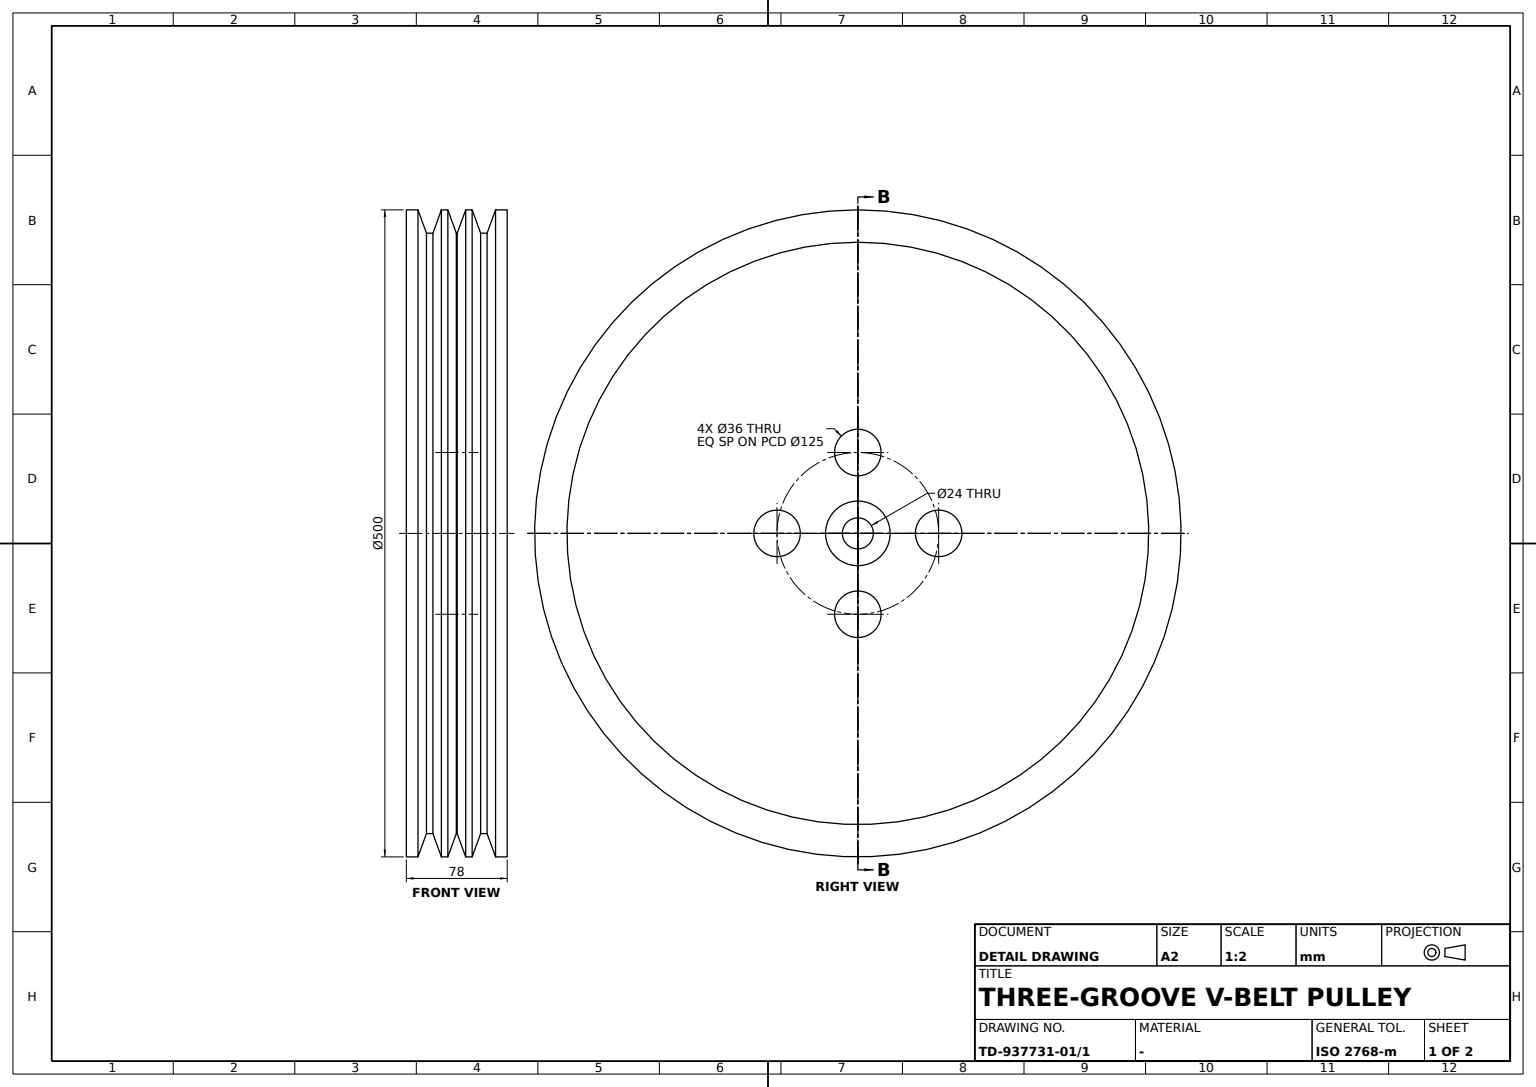
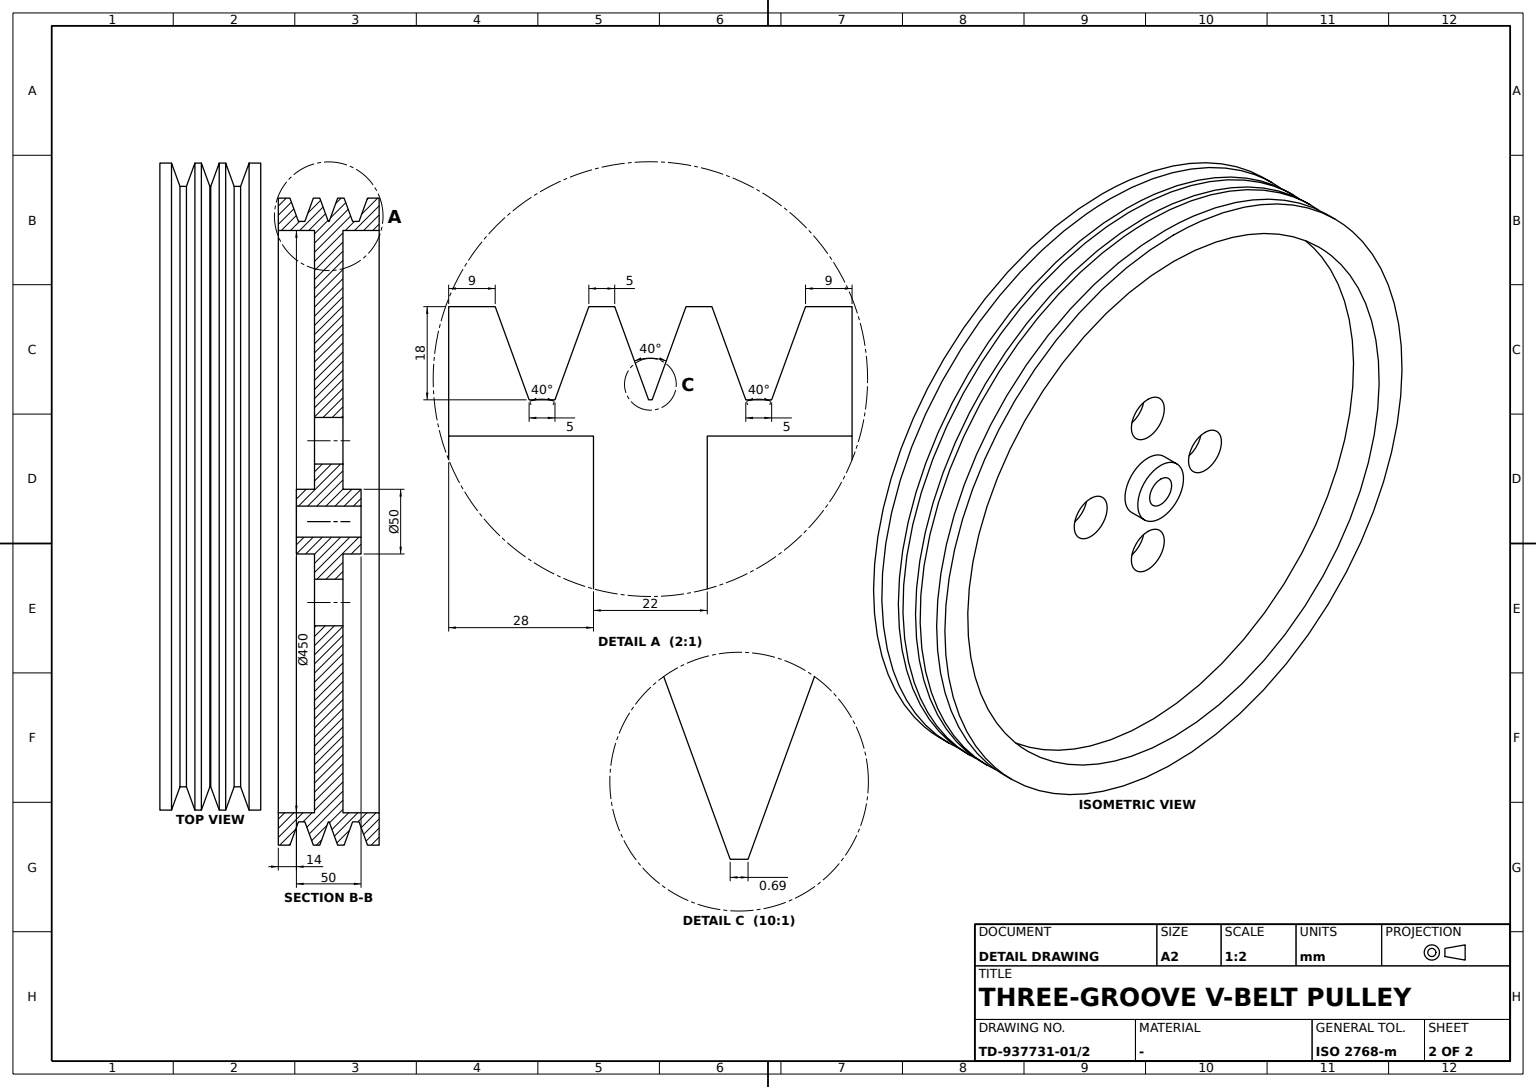
ISO-10303-21;
HEADER;
FILE_DESCRIPTION((''),'2;1');
FILE_NAME('','',(''),(''),'','','');
FILE_SCHEMA(('AUTOMOTIVE_DESIGN'));
ENDSEC;
DATA;
#1=APPLICATION_CONTEXT('');
#2=PRODUCT_CONTEXT('',#1,'mechanical');
#3=PRODUCT('','','',(#2));
#4=PRODUCT_DEFINITION_FORMATION('','',#3);
#5=PRODUCT_DEFINITION_CONTEXT('',#1,'design');
#6=PRODUCT_DEFINITION('','',#4,#5);
#7=PRODUCT_DEFINITION_SHAPE('','',#6);
#8=(LENGTH_UNIT()NAMED_UNIT(*)SI_UNIT(.MILLI.,.METRE.));
#9=(NAMED_UNIT(*)PLANE_ANGLE_UNIT()SI_UNIT($,.RADIAN.));
#10=(NAMED_UNIT(*)SI_UNIT($,.STERADIAN.)SOLID_ANGLE_UNIT());
#11=UNCERTAINTY_MEASURE_WITH_UNIT(LENGTH_MEASURE(0.005),#8,'distance_accuracy_value','');
#12=(GEOMETRIC_REPRESENTATION_CONTEXT(3)GLOBAL_UNCERTAINTY_ASSIGNED_CONTEXT((#11))GLOBAL_UNIT_ASSIGNED_CONTEXT((#8,#9,#10))REPRESENTATION_CONTEXT('',''));
#13=CARTESIAN_POINT('',(0.,6.897072,250.));
#14=VERTEX_POINT('',#13);
#15=CARTESIAN_POINT('',(0.,6.897072,0.));
#16=DIRECTION('',(0.,1.,0.));
#17=DIRECTION('',(0.,0.,1.));
#18=AXIS2_PLACEMENT_3D('',#15,#16,#17);
#19=CIRCLE('',#18,250.);
#20=EDGE_CURVE('',#14,#14,#19,.T.);
#21=ORIENTED_EDGE('',*,*,#20,.F.);
#22=EDGE_LOOP('',(#21));
#23=FACE_BOUND('',#22,.T.);
#24=CARTESIAN_POINT('',(0.,0.345607,232.));
#25=VERTEX_POINT('',#24);
#26=CARTESIAN_POINT('',(0.,0.345607,0.));
#27=AXIS2_PLACEMENT_3D('',#26,#16,#17);
#28=CIRCLE('',#27,232.);
#29=EDGE_CURVE('',#25,#25,#28,.T.);
#30=ORIENTED_EDGE('',*,*,#29,.T.);
#31=EDGE_LOOP('',(#30));
#32=FACE_BOUND('',#31,.T.);
#33=DIRECTION('',(1.,0.,0.));
#34=AXIS2_PLACEMENT_3D('',#26,#16,#33);
#35=CONICAL_SURFACE('',#34,232.,1.221730476);
#36=ADVANCED_FACE('',(#23,#32),#35,.T.);
#37=CARTESIAN_POINT('',(0.,25.,12.));
#38=VERTEX_POINT('',#37);
#39=CARTESIAN_POINT('',(0.,25.,0.));
#40=AXIS2_PLACEMENT_3D('',#39,#16,#17);
#41=CIRCLE('',#40,12.);
#42=EDGE_CURVE('',#38,#38,#41,.T.);
#43=ORIENTED_EDGE('',*,*,#42,.F.);
#44=EDGE_LOOP('',(#43));
#45=FACE_BOUND('',#44,.T.);
#46=CARTESIAN_POINT('',(0.,25.,25.));
#47=VERTEX_POINT('',#46);
#48=CIRCLE('',#40,25.);
#49=EDGE_CURVE('',#47,#47,#48,.T.);
#50=ORIENTED_EDGE('',*,*,#49,.T.);
#51=EDGE_LOOP('',(#50));
#52=FACE_BOUND('',#51,.T.);
#53=AXIS2_PLACEMENT_3D('',#46,#16,#33);
#54=PLANE('',#53);
#55=ADVANCED_FACE('',(#45,#52),#54,.T.);
#56=CARTESIAN_POINT('',(0.,18.448536,-232.));
#57=VERTEX_POINT('',#56);
#58=CARTESIAN_POINT('',(0.,18.448536,0.));
#59=DIRECTION('',(0.,-1.,0.));
#60=DIRECTION('',(0.,0.,-1.));
#61=AXIS2_PLACEMENT_3D('',#58,#59,#60);
#62=CIRCLE('',#61,232.);
#63=EDGE_CURVE('',#57,#57,#62,.F.);
#64=ORIENTED_EDGE('',*,*,#63,.F.);
#65=EDGE_LOOP('',(#64));
#66=FACE_BOUND('',#65,.T.);
#67=CARTESIAN_POINT('',(0.,11.897072,-250.));
#68=VERTEX_POINT('',#67);
#69=CARTESIAN_POINT('',(0.,11.897072,0.));
#70=AXIS2_PLACEMENT_3D('',#69,#59,#60);
#71=CIRCLE('',#70,250.);
#72=EDGE_CURVE('',#68,#68,#71,.F.);
#73=ORIENTED_EDGE('',*,*,#72,.T.);
#74=EDGE_LOOP('',(#73));
#75=FACE_BOUND('',#74,.T.);
#76=AXIS2_PLACEMENT_3D('',#58,#59,#33);
#77=CONICAL_SURFACE('',#76,232.,1.221730476);
#78=ADVANCED_FACE('',(#66,#75),#77,.T.);
#79=CARTESIAN_POINT('',(0.,30.,250.));
#80=VERTEX_POINT('',#79);
#81=CARTESIAN_POINT('',(0.,30.,0.));
#82=AXIS2_PLACEMENT_3D('',#81,#16,#17);
#83=CIRCLE('',#82,250.);
#84=EDGE_CURVE('',#80,#80,#83,.T.);
#85=ORIENTED_EDGE('',*,*,#84,.T.);
#86=EDGE_LOOP('',(#85));
#87=FACE_BOUND('',#86,.T.);
#88=CARTESIAN_POINT('',(0.,39.,250.));
#89=VERTEX_POINT('',#88);
#90=CARTESIAN_POINT('',(0.,39.,0.));
#91=AXIS2_PLACEMENT_3D('',#90,#16,#17);
#92=CIRCLE('',#91,250.);
#93=EDGE_CURVE('',#89,#89,#92,.T.);
#94=ORIENTED_EDGE('',*,*,#93,.F.);
#95=EDGE_LOOP('',(#94));
#96=FACE_BOUND('',#95,.T.);
#97=CARTESIAN_POINT('',(0.,0.,0.));
#98=AXIS2_PLACEMENT_3D('',#97,#16,#33);
#99=CYLINDRICAL_SURFACE('',#98,250.);
#100=ADVANCED_FACE('',(#87,#96),#99,.T.);
#101=ORIENTED_EDGE('',*,*,#42,.T.);
#102=EDGE_LOOP('',(#101));
#103=FACE_BOUND('',#102,.T.);
#104=CARTESIAN_POINT('',(0.,-25.,12.));
#105=VERTEX_POINT('',#104);
#106=CARTESIAN_POINT('',(0.,-25.,0.));
#107=AXIS2_PLACEMENT_3D('',#106,#16,#17);
#108=CIRCLE('',#107,12.);
#109=EDGE_CURVE('',#105,#105,#108,.T.);
#110=ORIENTED_EDGE('',*,*,#109,.F.);
#111=EDGE_LOOP('',(#110));
#112=FACE_BOUND('',#111,.T.);
#113=CYLINDRICAL_SURFACE('',#98,12.);
#114=ADVANCED_FACE('',(#103,#112),#113,.F.);
#115=CARTESIAN_POINT('',(0.,-11.,225.));
#116=VERTEX_POINT('',#115);
#117=CARTESIAN_POINT('',(0.,-11.,0.));
#118=AXIS2_PLACEMENT_3D('',#117,#16,#17);
#119=CIRCLE('',#118,225.);
#120=EDGE_CURVE('',#116,#116,#119,.T.);
#121=ORIENTED_EDGE('',*,*,#120,.T.);
#122=EDGE_LOOP('',(#121));
#123=FACE_BOUND('',#122,.T.);
#124=CARTESIAN_POINT('',(0.,-39.,225.));
#125=VERTEX_POINT('',#124);
#126=CARTESIAN_POINT('',(0.,-39.,0.));
#127=AXIS2_PLACEMENT_3D('',#126,#16,#17);
#128=CIRCLE('',#127,225.);
#129=EDGE_CURVE('',#125,#125,#128,.T.);
#130=ORIENTED_EDGE('',*,*,#129,.F.);
#131=EDGE_LOOP('',(#130));
#132=FACE_BOUND('',#131,.T.);
#133=CYLINDRICAL_SURFACE('',#98,225.);
#134=ADVANCED_FACE('',(#123,#132),#133,.F.);
#135=CARTESIAN_POINT('',(0.,-18.448536,232.));
#136=VERTEX_POINT('',#135);
#137=CARTESIAN_POINT('',(0.,-18.448536,0.));
#138=AXIS2_PLACEMENT_3D('',#137,#16,#17);
#139=CIRCLE('',#138,232.);
#140=EDGE_CURVE('',#136,#136,#139,.T.);
#141=ORIENTED_EDGE('',*,*,#140,.T.);
#142=EDGE_LOOP('',(#141));
#143=FACE_BOUND('',#142,.T.);
#144=CARTESIAN_POINT('',(0.,-11.897072,250.));
#145=VERTEX_POINT('',#144);
#146=CARTESIAN_POINT('',(0.,-11.897072,0.));
#147=AXIS2_PLACEMENT_3D('',#146,#16,#17);
#148=CIRCLE('',#147,250.);
#149=EDGE_CURVE('',#145,#145,#148,.T.);
#150=ORIENTED_EDGE('',*,*,#149,.F.);
#151=EDGE_LOOP('',(#150));
#152=FACE_BOUND('',#151,.T.);
#153=AXIS2_PLACEMENT_3D('',#137,#16,#33);
#154=CONICAL_SURFACE('',#153,232.,1.221730476);
#155=ADVANCED_FACE('',(#143,#152),#154,.T.);
#156=CARTESIAN_POINT('',(0.,-30.,-250.));
#157=VERTEX_POINT('',#156);
#158=CARTESIAN_POINT('',(0.,-30.,0.));
#159=AXIS2_PLACEMENT_3D('',#158,#59,#60);
#160=CIRCLE('',#159,250.);
#161=EDGE_CURVE('',#157,#157,#160,.F.);
#162=ORIENTED_EDGE('',*,*,#161,.T.);
#163=EDGE_LOOP('',(#162));
#164=FACE_BOUND('',#163,.T.);
#165=CARTESIAN_POINT('',(0.,-23.448536,-232.));
#166=VERTEX_POINT('',#165);
#167=CARTESIAN_POINT('',(0.,-23.448536,0.));
#168=AXIS2_PLACEMENT_3D('',#167,#59,#60);
#169=CIRCLE('',#168,232.);
#170=EDGE_CURVE('',#166,#166,#169,.F.);
#171=ORIENTED_EDGE('',*,*,#170,.F.);
#172=EDGE_LOOP('',(#171));
#173=FACE_BOUND('',#172,.T.);
#174=AXIS2_PLACEMENT_3D('',#167,#59,#33);
#175=CONICAL_SURFACE('',#174,232.,1.221730476);
#176=ADVANCED_FACE('',(#164,#173),#175,.T.);
#177=CARTESIAN_POINT('',(0.,-0.345607,-232.));
#178=VERTEX_POINT('',#177);
#179=CARTESIAN_POINT('',(0.,-0.345607,0.));
#180=AXIS2_PLACEMENT_3D('',#179,#59,#60);
#181=CIRCLE('',#180,232.);
#182=EDGE_CURVE('',#178,#178,#181,.F.);
#183=ORIENTED_EDGE('',*,*,#182,.F.);
#184=EDGE_LOOP('',(#183));
#185=FACE_BOUND('',#184,.T.);
#186=CARTESIAN_POINT('',(0.,-6.897072,-250.));
#187=VERTEX_POINT('',#186);
#188=CARTESIAN_POINT('',(0.,-6.897072,0.));
#189=AXIS2_PLACEMENT_3D('',#188,#59,#60);
#190=CIRCLE('',#189,250.);
#191=EDGE_CURVE('',#187,#187,#190,.F.);
#192=ORIENTED_EDGE('',*,*,#191,.T.);
#193=EDGE_LOOP('',(#192));
#194=FACE_BOUND('',#193,.T.);
#195=AXIS2_PLACEMENT_3D('',#179,#59,#33);
#196=CONICAL_SURFACE('',#195,232.,1.221730476);
#197=ADVANCED_FACE('',(#185,#194),#196,.T.);
#198=CARTESIAN_POINT('',(0.,-11.,-44.5));
#199=VERTEX_POINT('',#198);
#200=CARTESIAN_POINT('',(0.,-11.,-62.5));
#201=AXIS2_PLACEMENT_3D('',#200,#16,#17);
#202=CIRCLE('',#201,18.);
#203=EDGE_CURVE('',#199,#199,#202,.T.);
#204=ORIENTED_EDGE('',*,*,#203,.F.);
#205=EDGE_LOOP('',(#204));
#206=FACE_BOUND('',#205,.T.);
#207=CARTESIAN_POINT('',(0.,11.,-44.5));
#208=VERTEX_POINT('',#207);
#209=CARTESIAN_POINT('',(0.,11.,-62.5));
#210=AXIS2_PLACEMENT_3D('',#209,#16,#17);
#211=CIRCLE('',#210,18.);
#212=EDGE_CURVE('',#208,#208,#211,.T.);
#213=ORIENTED_EDGE('',*,*,#212,.T.);
#214=EDGE_LOOP('',(#213));
#215=FACE_BOUND('',#214,.T.);
#216=CARTESIAN_POINT('',(0.,-32.5,-62.5));
#217=DIRECTION('',(-1.,0.,0.));
#218=AXIS2_PLACEMENT_3D('',#216,#16,#217);
#219=CYLINDRICAL_SURFACE('',#218,18.);
#220=ADVANCED_FACE('',(#206,#215),#219,.F.);
#221=CARTESIAN_POINT('',(0.,11.,25.));
#222=VERTEX_POINT('',#221);
#223=CARTESIAN_POINT('',(0.,11.,0.));
#224=AXIS2_PLACEMENT_3D('',#223,#16,#17);
#225=CIRCLE('',#224,25.);
#226=EDGE_CURVE('',#222,#222,#225,.T.);
#227=ORIENTED_EDGE('',*,*,#226,.T.);
#228=EDGE_LOOP('',(#227));
#229=FACE_BOUND('',#228,.T.);
#230=ORIENTED_EDGE('',*,*,#49,.F.);
#231=EDGE_LOOP('',(#230));
#232=FACE_BOUND('',#231,.T.);
#233=CYLINDRICAL_SURFACE('',#98,25.);
#234=ADVANCED_FACE('',(#229,#232),#233,.T.);
#235=ORIENTED_EDGE('',*,*,#84,.F.);
#236=EDGE_LOOP('',(#235));
#237=FACE_BOUND('',#236,.T.);
#238=CARTESIAN_POINT('',(0.,23.448536,232.));
#239=VERTEX_POINT('',#238);
#240=CARTESIAN_POINT('',(0.,23.448536,0.));
#241=AXIS2_PLACEMENT_3D('',#240,#16,#17);
#242=CIRCLE('',#241,232.);
#243=EDGE_CURVE('',#239,#239,#242,.T.);
#244=ORIENTED_EDGE('',*,*,#243,.T.);
#245=EDGE_LOOP('',(#244));
#246=FACE_BOUND('',#245,.T.);
#247=AXIS2_PLACEMENT_3D('',#240,#16,#33);
#248=CONICAL_SURFACE('',#247,232.,1.221730476);
#249=ADVANCED_FACE('',(#237,#246),#248,.T.);
#250=CARTESIAN_POINT('',(-62.5,11.,18.));
#251=VERTEX_POINT('',#250);
#252=CARTESIAN_POINT('',(-62.5,11.,0.));
#253=AXIS2_PLACEMENT_3D('',#252,#16,#17);
#254=CIRCLE('',#253,18.);
#255=EDGE_CURVE('',#251,#251,#254,.T.);
#256=ORIENTED_EDGE('',*,*,#255,.T.);
#257=EDGE_LOOP('',(#256));
#258=FACE_BOUND('',#257,.T.);
#259=CARTESIAN_POINT('',(-62.5,-11.,18.));
#260=VERTEX_POINT('',#259);
#261=CARTESIAN_POINT('',(-62.5,-11.,0.));
#262=AXIS2_PLACEMENT_3D('',#261,#16,#17);
#263=CIRCLE('',#262,18.);
#264=EDGE_CURVE('',#260,#260,#263,.T.);
#265=ORIENTED_EDGE('',*,*,#264,.F.);
#266=EDGE_LOOP('',(#265));
#267=FACE_BOUND('',#266,.T.);
#268=CARTESIAN_POINT('',(-62.5,-32.5,0.));
#269=AXIS2_PLACEMENT_3D('',#268,#16,#217);
#270=CYLINDRICAL_SURFACE('',#269,18.);
#271=ADVANCED_FACE('',(#258,#267),#270,.F.);
#272=ORIENTED_EDGE('',*,*,#20,.T.);
#273=EDGE_LOOP('',(#272));
#274=FACE_BOUND('',#273,.T.);
#275=ORIENTED_EDGE('',*,*,#72,.F.);
#276=EDGE_LOOP('',(#275));
#277=FACE_BOUND('',#276,.T.);
#278=ADVANCED_FACE('',(#274,#277),#99,.T.);
#279=CARTESIAN_POINT('',(0.,11.,225.));
#280=VERTEX_POINT('',#279);
#281=CIRCLE('',#224,225.);
#282=EDGE_CURVE('',#280,#280,#281,.T.);
#283=ORIENTED_EDGE('',*,*,#282,.T.);
#284=EDGE_LOOP('',(#283));
#285=FACE_BOUND('',#284,.T.);
#286=CARTESIAN_POINT('',(62.5,11.,18.));
#287=VERTEX_POINT('',#286);
#288=CARTESIAN_POINT('',(62.5,11.,0.));
#289=AXIS2_PLACEMENT_3D('',#288,#16,#17);
#290=CIRCLE('',#289,18.);
#291=EDGE_CURVE('',#287,#287,#290,.T.);
#292=ORIENTED_EDGE('',*,*,#291,.F.);
#293=EDGE_LOOP('',(#292));
#294=FACE_BOUND('',#293,.T.);
#295=CARTESIAN_POINT('',(0.,11.,80.5));
#296=VERTEX_POINT('',#295);
#297=CARTESIAN_POINT('',(0.,11.,62.5));
#298=AXIS2_PLACEMENT_3D('',#297,#16,#17);
#299=CIRCLE('',#298,18.);
#300=EDGE_CURVE('',#296,#296,#299,.T.);
#301=ORIENTED_EDGE('',*,*,#300,.F.);
#302=EDGE_LOOP('',(#301));
#303=FACE_BOUND('',#302,.T.);
#304=ORIENTED_EDGE('',*,*,#212,.F.);
#305=EDGE_LOOP('',(#304));
#306=FACE_BOUND('',#305,.T.);
#307=ORIENTED_EDGE('',*,*,#255,.F.);
#308=EDGE_LOOP('',(#307));
#309=FACE_BOUND('',#308,.T.);
#310=ORIENTED_EDGE('',*,*,#226,.F.);
#311=EDGE_LOOP('',(#310));
#312=FACE_BOUND('',#311,.T.);
#313=AXIS2_PLACEMENT_3D('',#279,#16,#33);
#314=PLANE('',#313);
#315=ADVANCED_FACE('',(#285,#294,#303,#306,#309,#312),#314,.T.);
#316=ORIENTED_EDGE('',*,*,#149,.T.);
#317=EDGE_LOOP('',(#316));
#318=FACE_BOUND('',#317,.T.);
#319=ORIENTED_EDGE('',*,*,#191,.F.);
#320=EDGE_LOOP('',(#319));
#321=FACE_BOUND('',#320,.T.);
#322=ADVANCED_FACE('',(#318,#321),#99,.T.);
#323=CARTESIAN_POINT('',(0.,39.,225.));
#324=VERTEX_POINT('',#323);
#325=CIRCLE('',#91,225.);
#326=EDGE_CURVE('',#324,#324,#325,.T.);
#327=ORIENTED_EDGE('',*,*,#326,.F.);
#328=EDGE_LOOP('',(#327));
#329=FACE_BOUND('',#328,.T.);
#330=ORIENTED_EDGE('',*,*,#93,.T.);
#331=EDGE_LOOP('',(#330));
#332=FACE_BOUND('',#331,.T.);
#333=AXIS2_PLACEMENT_3D('',#88,#16,#33);
#334=PLANE('',#333);
#335=ADVANCED_FACE('',(#329,#332),#334,.T.);
#336=ORIENTED_EDGE('',*,*,#129,.T.);
#337=EDGE_LOOP('',(#336));
#338=FACE_BOUND('',#337,.T.);
#339=CARTESIAN_POINT('',(0.,-39.,250.));
#340=VERTEX_POINT('',#339);
#341=CIRCLE('',#127,250.);
#342=EDGE_CURVE('',#340,#340,#341,.T.);
#343=ORIENTED_EDGE('',*,*,#342,.F.);
#344=EDGE_LOOP('',(#343));
#345=FACE_BOUND('',#344,.T.);
#346=AXIS2_PLACEMENT_3D('',#339,#16,#33);
#347=PLANE('',#346);
#348=ADVANCED_FACE('',(#338,#345),#347,.F.);
#349=ORIENTED_EDGE('',*,*,#300,.T.);
#350=EDGE_LOOP('',(#349));
#351=FACE_BOUND('',#350,.T.);
#352=CARTESIAN_POINT('',(0.,-11.,80.5));
#353=VERTEX_POINT('',#352);
#354=CARTESIAN_POINT('',(0.,-11.,62.5));
#355=AXIS2_PLACEMENT_3D('',#354,#16,#17);
#356=CIRCLE('',#355,18.);
#357=EDGE_CURVE('',#353,#353,#356,.T.);
#358=ORIENTED_EDGE('',*,*,#357,.F.);
#359=EDGE_LOOP('',(#358));
#360=FACE_BOUND('',#359,.T.);
#361=CARTESIAN_POINT('',(0.,-32.5,62.5));
#362=AXIS2_PLACEMENT_3D('',#361,#16,#217);
#363=CYLINDRICAL_SURFACE('',#362,18.);
#364=ADVANCED_FACE('',(#351,#360),#363,.F.);
#365=ORIENTED_EDGE('',*,*,#140,.F.);
#366=EDGE_LOOP('',(#365));
#367=FACE_BOUND('',#366,.T.);
#368=ORIENTED_EDGE('',*,*,#170,.T.);
#369=EDGE_LOOP('',(#368));
#370=FACE_BOUND('',#369,.T.);
#371=CYLINDRICAL_SURFACE('',#98,232.);
#372=ADVANCED_FACE('',(#367,#370),#371,.T.);
#373=ORIENTED_EDGE('',*,*,#291,.T.);
#374=EDGE_LOOP('',(#373));
#375=FACE_BOUND('',#374,.T.);
#376=CARTESIAN_POINT('',(62.5,-11.,18.));
#377=VERTEX_POINT('',#376);
#378=CARTESIAN_POINT('',(62.5,-11.,0.));
#379=AXIS2_PLACEMENT_3D('',#378,#16,#17);
#380=CIRCLE('',#379,18.);
#381=EDGE_CURVE('',#377,#377,#380,.T.);
#382=ORIENTED_EDGE('',*,*,#381,.F.);
#383=EDGE_LOOP('',(#382));
#384=FACE_BOUND('',#383,.T.);
#385=CARTESIAN_POINT('',(62.5,-32.5,0.));
#386=AXIS2_PLACEMENT_3D('',#385,#16,#217);
#387=CYLINDRICAL_SURFACE('',#386,18.);
#388=ADVANCED_FACE('',(#375,#384),#387,.F.);
#389=ORIENTED_EDGE('',*,*,#342,.T.);
#390=EDGE_LOOP('',(#389));
#391=FACE_BOUND('',#390,.T.);
#392=ORIENTED_EDGE('',*,*,#161,.F.);
#393=EDGE_LOOP('',(#392));
#394=FACE_BOUND('',#393,.T.);
#395=ADVANCED_FACE('',(#391,#394),#99,.T.);
#396=CARTESIAN_POINT('',(0.,-11.,25.));
#397=VERTEX_POINT('',#396);
#398=CIRCLE('',#118,25.);
#399=EDGE_CURVE('',#397,#397,#398,.T.);
#400=ORIENTED_EDGE('',*,*,#399,.F.);
#401=EDGE_LOOP('',(#400));
#402=FACE_BOUND('',#401,.T.);
#403=CARTESIAN_POINT('',(0.,-25.,25.));
#404=VERTEX_POINT('',#403);
#405=CIRCLE('',#107,25.);
#406=EDGE_CURVE('',#404,#404,#405,.T.);
#407=ORIENTED_EDGE('',*,*,#406,.T.);
#408=EDGE_LOOP('',(#407));
#409=FACE_BOUND('',#408,.T.);
#410=ADVANCED_FACE('',(#402,#409),#233,.T.);
#411=ORIENTED_EDGE('',*,*,#63,.T.);
#412=EDGE_LOOP('',(#411));
#413=FACE_BOUND('',#412,.T.);
#414=ORIENTED_EDGE('',*,*,#243,.F.);
#415=EDGE_LOOP('',(#414));
#416=FACE_BOUND('',#415,.T.);
#417=ADVANCED_FACE('',(#413,#416),#371,.T.);
#418=ORIENTED_EDGE('',*,*,#282,.F.);
#419=EDGE_LOOP('',(#418));
#420=FACE_BOUND('',#419,.T.);
#421=ORIENTED_EDGE('',*,*,#326,.T.);
#422=EDGE_LOOP('',(#421));
#423=FACE_BOUND('',#422,.T.);
#424=ADVANCED_FACE('',(#420,#423),#133,.F.);
#425=ORIENTED_EDGE('',*,*,#29,.F.);
#426=EDGE_LOOP('',(#425));
#427=FACE_BOUND('',#426,.T.);
#428=ORIENTED_EDGE('',*,*,#182,.T.);
#429=EDGE_LOOP('',(#428));
#430=FACE_BOUND('',#429,.T.);
#431=ADVANCED_FACE('',(#427,#430),#371,.T.);
#432=ORIENTED_EDGE('',*,*,#406,.F.);
#433=EDGE_LOOP('',(#432));
#434=FACE_BOUND('',#433,.T.);
#435=ORIENTED_EDGE('',*,*,#109,.T.);
#436=EDGE_LOOP('',(#435));
#437=FACE_BOUND('',#436,.T.);
#438=AXIS2_PLACEMENT_3D('',#403,#16,#33);
#439=PLANE('',#438);
#440=ADVANCED_FACE('',(#434,#437),#439,.F.);
#441=ORIENTED_EDGE('',*,*,#264,.T.);
#442=EDGE_LOOP('',(#441));
#443=FACE_BOUND('',#442,.T.);
#444=ORIENTED_EDGE('',*,*,#120,.F.);
#445=EDGE_LOOP('',(#444));
#446=FACE_BOUND('',#445,.T.);
#447=ORIENTED_EDGE('',*,*,#399,.T.);
#448=EDGE_LOOP('',(#447));
#449=FACE_BOUND('',#448,.T.);
#450=ORIENTED_EDGE('',*,*,#357,.T.);
#451=EDGE_LOOP('',(#450));
#452=FACE_BOUND('',#451,.T.);
#453=ORIENTED_EDGE('',*,*,#203,.T.);
#454=EDGE_LOOP('',(#453));
#455=FACE_BOUND('',#454,.T.);
#456=ORIENTED_EDGE('',*,*,#381,.T.);
#457=EDGE_LOOP('',(#456));
#458=FACE_BOUND('',#457,.T.);
#459=AXIS2_PLACEMENT_3D('',#115,#16,#33);
#460=PLANE('',#459);
#461=ADVANCED_FACE('',(#443,#446,#449,#452,#455,#458),#460,.F.);
#462=CLOSED_SHELL('',(#36,#55,#78,#100,#114,#134,#155,#176,#197,#220,#234,#249,#271,#278,#315,#322,#335,#348,#364,#372,#388,#395,#410,#417,#424,#431,#440,#461));
#463=MANIFOLD_SOLID_BREP('',#462);
#464=ADVANCED_BREP_SHAPE_REPRESENTATION('',(#463),#12);
#465=SHAPE_DEFINITION_REPRESENTATION(#7,#464);
ENDSEC;
END-ISO-10303-21;
